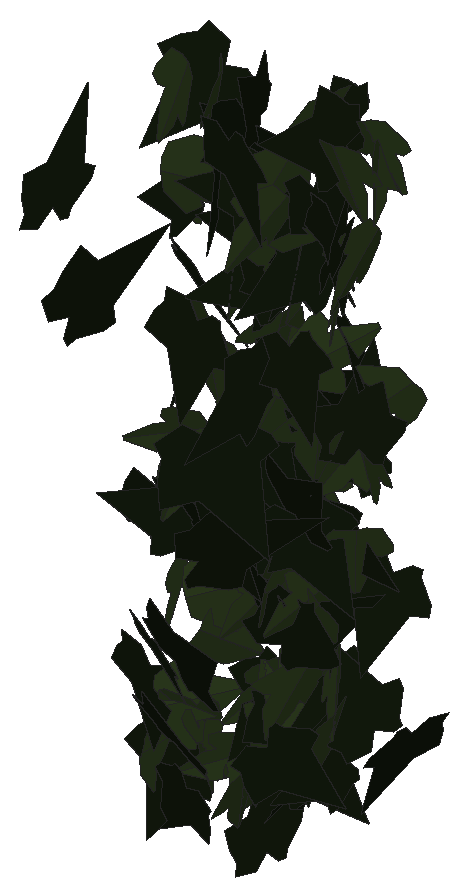
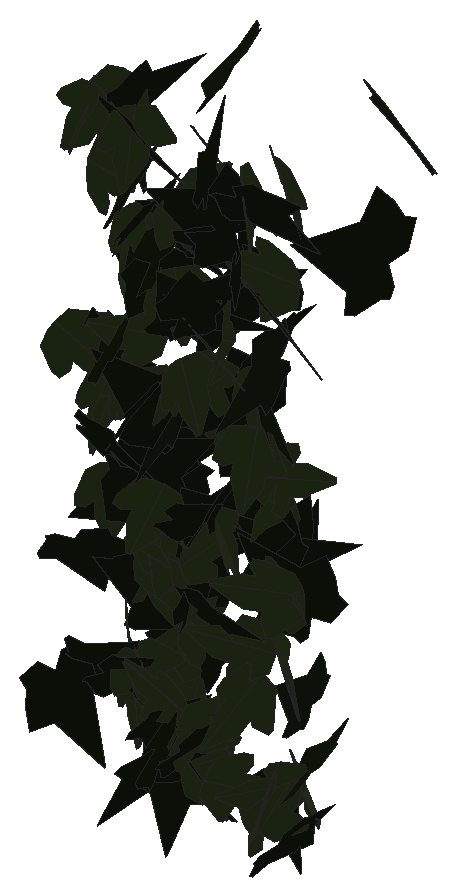
# SketchUp Ruby script. Lengths in inches.
U = 1.inch
M = Sketchup.active_model
def pt(a) = Geom::Point3d.new(a.map { |v| v * U })
def face(e, loops, mat)
  f = e.add_face(loops[0].map { |a| pt(a) })
  loops[1..].each { |l| e.add_face(l.map { |a| pt(a) }).erase! }
  f.material = f.back_material = mat if mat
  f
end
# faces: each face lists its corners as indices into pts; further lists are holes
def faces(e, pts, list, mat = nil) = list.each { |f| face(e, (f[0].is_a?(Array) ? f : [f]).map { |l| l.map { |i| pts[i] } }, mat) }
# xy, xz, yz: faces in a plane at the given z, y or x. An outline is a flat list of corners, or four numbers for a rectangle; further outlines are holes
def ring(l) = l.size == 4 ? [[l[0], l[1]], [l[2], l[1]], [l[2], l[3]], [l[0], l[3]]] : l.each_slice(2).to_a
def flat(e, list, mat, &to3) = list.each { |f| face(e, (f[0].is_a?(Array) ? f : [f]).map { |l| ring(l).map { |u, v| to3.(u, v) } }, mat) }
def xy(e, z, list, mat = nil) = flat(e, list, mat) { |x, y| [x, y, z] }
def xz(e, y, list, mat = nil) = flat(e, list, mat) { |x, z| [x, y, z] }
def yz(e, x, list, mat = nil) = flat(e, list, mat) { |y, z| [x, y, z] }
def lines(e, pts, list) = list.each { |a, b| e.add_line(pt(pts[a]), pt(pts[b])) }
# prism: a flat outline (further loops are holes) pulled along v
def prism(e, loops, v, mat = nil)
  f = face(e, loops, mat); d = Geom::Vector3d.new(v.map { |x| x * U })
  f.pushpull(f.normal.samedirection?(d) ? d.length : -d.length)
end
def box(e, o, s, mat = nil) = prism(e, [[o, [o[0] + s[0], o[1], o[2]], [o[0] + s[0], o[1] + s[1], o[2]], [o[0], o[1] + s[1], o[2]]]], [0, 0, s[2]], mat)
def at(x, y, z, deg = 0) = Geom::Transformation.translation(pt([x, y, z])) * Geom::Transformation.rotation(ORIGIN, Z_AXIS, deg.degrees)
def axes(o, x, y, z) = Geom::Transformation.new([*x, 0, *y, 0, *z, 0, *pt(o).to_a, 1])
def part(name) = M.definitions.add(name)
# library, detail: a bought-in or finely detailed component or shape, given as its bounding box
def library(name, o, s) = part(name).tap { |d| box(d.entities, o, s) }
def detail(e, o, s) = box(e.add_group.entities, o, s)
def put(e, d, t, mat = nil) = e.add_instance(d, t).tap { |i| i.material = mat if mat }
def group(e, t, mat = nil) = e.add_group.tap { |g| g.transformation = t; g.material = mat if mat }.entities
root = M.entities
M.materials.add("efeu1").color = [18, 25, 13]
M.materials.add("efeu2").color = [43, 57, 29]
c1 = part("ivyleaf_9")
p = [[1.54,2.16,1.25],[1.36,2.04,1.19],[-0.21,0.99,0.68],[-0.71,1.11,0.82],[-0.85,0.86,0.67],[-0.8,0.17,0.21],
  [-0.9,-0.01,0.1],[-0.67,-0.16,-0.02],[-0.08,-0.08,-0.05],[-0.03,-0.6,-0.4],[0.65,-0.88,-0.66],[0.83,-0.6,-0.49],
  [1.29,-0.42,-0.43],[1.8125,-0.07,-0.26],[1.21,0.44,0.15]]
faces(c1.entities,p,[[0,1,2,3,4,5,6,7,8,9,10,11,12,13,14]],"efeu1")
c2 = part("ivyleaf_10")
p = [[0,0.5,-0.03],[-0.0625,2.02,-0.43],[-0.19,2.01,-0.46],[-0.54,1.05,-0.29],[-0.52,0.625,-0.18],[-0.83,0.76,-0.28],
  [-1.16,0.64,-0.33],[-1.15,0.33,-0.24],[-0.77,-0.39,0.02],[-0.3,-0.51,0.16],[0.04,-0.48,0.23],[-0.02,2.01,-0.4375],
  [-0.06,2.01,-0.43],[0.04,-0.49,0.23],[0.67,-0.49,0.14],[1.38,0.36,-0.2],[1.375,0.51,-0.24],[0.81,0.65,-0.19],
  [0.62,0.59,-0.15],[0.6,1.09,-0.28],[0.5,1.23,-0.31]]
faces(c2.entities,p,[[0,1,2,3,4,5,6,7,8,9,10],[11,12,0,13,14,15,16,17,18,19,20]],"efeu2")
put(root,c1,axes([542.46,125.34,201.33],[-0.99662,0.33655,-0.15122],[0.14199,-0.05215,-1.05191],[-0.34055,-1.00668,0.00394]))
put(root,c1,axes([538.84,126.51,189.16],[0.8472,-0.56615,0.10588],[-0.08782,0.05915,1.01896],[-0.56923,-0.85174,0.00038]))
put(root,c1,axes([535.7,125.54,204.25],[-0.88917,0.67387,-0.10406],[-0.08581,0.05905,1.11567],[0.67644,0.89329,0.00475]))
put(root,c1,axes([540.1875,126.3,198.45],[-0.02484,-0.85792,-0.79296],[0.14605,0.78464,-0.85349],[1.15909,-0.11726,0.09055]))
put(root,c1,axes([538.32,127.29,190.98],[-0.04579,-0.29377,1.10403],[0.68746,-0.88957,-0.20819],[0.91246,0.65547,0.21226]))
put(root,c1,axes([535.68,126.37,200.66],[0.09702,0.07319,1.16134],[0.78915,0.8523,-0.11964],[-0.85517,0.7948,0.02135]))
put(root,c1,axes([539.65,126.72,194.68],[0.39362,0.23601,1.0665],[0.91867,0.54173,-0.45895],[-0.5909,0.99945,-0.00309]))
put(root,c1,axes([539.36,128.17,206.05],[0.42505,-0.88524,0.22608],[0.10685,-0.19947,-0.98195],[0.90738,0.43817,0.00972]))
put(root,c1,axes([540.29,128.63,188.47],[0.02358,-0.21935,-0.82404],[0.27211,0.78319,-0.20069],[0.80815,-0.25731,0.09162]))
put(root,c2,axes([539.11,128.93,187.01],[0.06972,-0.81984,-0.18916],[-0.01731,0.18837,-0.8228],[0.8412,0.07183,-0.00125]))
put(root,c1,axes([540.54,129.16,200.02],[0.08511,-0.8096,-0.26487],[-0.02314,0.26389,-0.81405],[0.85151,0.08809,0.00435]))
put(root,c1,axes([536.93,129.78,199.24],[-0.02769,-0.95204,0.27297],[-0.01795,-0.27255,-0.95239],[0.99024,-0.03156,-0.00964]))
put(root,c1,axes([536.92,129.39,185.79],[0.32793,0.12421,-0.75032],[-0.71071,-0.24082,-0.35049],[-0.27073,0.78264,0.01124]))
put(root,c1,axes([540.08,129.92,194.74],[-0.28154,-0.08244,0.94768],[0.58247,-0.79632,0.10377],[0.75208,0.58587,0.27439]))
put(root,c1,axes([542,128.98,203.02],[0.13248,0.21807,0.82631],[-0.1013,0.83429,-0.20394],[-0.84858,-0.06555,0.15335]))
put(root,c2,axes([539.08,130.26,203.14],[-0.12291,-0.64575,0.69785],[-0.04154,-0.69934,-0.65444],[0.94988,-0.11414,0.06168]))
put(root,c2,axes([542.03,130.39,203.1],[0.14763,-0.60488,0.75555],[0.23882,-0.71789,-0.62139],[0.93792,0.278,0.0393]))
put(root,c2,axes([539.28,129.92,197.56],[-0.67822,-0.56031,0.38123],[-0.30162,-0.23343,-0.87966],[0.60688,-0.74218,-0.01114]))
put(root,c2,axes([535.17,130.08,186.01],[0.2974,-0.46163,-0.60165],[0.44807,-0.41442,0.53946],[-0.61181,-0.5279,0.10262]))
put(root,c1,axes([535.17,130.17,189.2],[0.36127,-0.5464,0.48417],[0.28485,-0.39189,-0.65481],[0.67218,0.45974,0.01727]))
put(root,c2,axes([536.34,130.23,194.875],[0.1111,0.59983,-0.55383],[-0.11032,-0.54278,-0.60999],[-0.80892,0.15641,0.00713]))
put(root,c1,axes([538.37,130.21,193.11],[0.34532,0.16862,0.86839],[-0.84103,-0.22643,0.3784],[0.27425,-0.90669,0.06699]))
put(root,c1,axes([536.37,130.16,193.15],[-0.29124,0.00633,0.77085],[-0.76742,-0.08043,-0.28928],[0.07301,-0.8201,0.03432]))
put(root,c2,axes([536.35,130.28,195.69],[0.01568,0.15758,-0.80777],[-0.7282,-0.37377,-0.08705],[-0.38345,0.71626,0.13228]))
put(root,c2,axes([539.22,130.32,193.16],[0.47656,-0.76573,0.36457],[0.19543,-0.30778,-0.90191],[0.82527,0.51506,0.00305]))
put(root,c1,axes([539.44,129.54,184.93],[-0.8793,0.36104,-0.12202],[-0.12025,0.02832,0.95034],[0.36163,0.88728,0.01932]))
put(root,c1,axes([540.16,129.96,194.58],[-0.21178,-0.51876,-0.81864],[0.42013,0.70598,-0.55606],[0.87336,-0.46541,0.06898]))
put(root,c1,axes([538.51,129.92,196.47],[0.03525,-0.68505,-0.71505],[0.12812,0.71265,-0.67643],[0.98192,-0.0684,0.11393]))
put(root,c1,axes([540.95,130.74,205.49],[-0.29247,-0.1571,0.84291],[-0.55236,-0.64666,-0.31218],[0.65581,-0.61471,0.11298]))
put(root,c2,axes([540.11,130.67,192.11],[-0.02903,-0.37937,0.73832],[-0.07834,-0.73422,-0.38035],[0.82638,-0.08293,-0.01012]))
put(root,c1,axes([535.86,130.36,193.2],[0.22248,-0.24255,0.75106],[0.55341,-0.50842,-0.32813],[0.56272,0.5959,0.02575]))
put(root,c1,axes([540.43,130.4,202.18],[-0.96021,-0.022,0.11467],[-0.11468,-0.00107,-0.96046],[0.02197,-0.96704,-0.00155]))
put(root,c2,axes([538.55,130.81,186.38],[0.02886,-0.1984,0.87429],[0.28414,-0.82763,-0.19719],[0.8503,0.2833,0.03622]))
put(root,c1,axes([540.74,130.7,202.98],[0.25081,-0.78857,0.41667],[0.09233,-0.40755,-0.82689],[0.88709,0.26538,-0.03174]))
put(root,c2,axes([541.44,130.12,205.51],[-0.91099,0.12476,-0.14051],[0.13928,-0.01856,-0.91949],[-0.12613,-0.92158,-0.0005]))
put(root,c2,axes([539.56,130.68,189.38],[-0.2199,-0.7841,0.39939],[-0.0943,-0.3883,-0.81425],[0.87489,-0.23893,0.01262]))
put(root,c2,axes([541.32,130.85,196.67],[0.12495,0.40976,-0.73646],[-0.27603,-0.68354,-0.42715],[-0.79629,0.30125,0.03251]))
put(root,c1,axes([541.21,130.47,187.64],[-0.8341,0.23111,0.14881],[-0.14103,0.04828,-0.86548],[-0.23593,-0.84589,-0.00874]))
put(root,c1,axes([534.47,131,187.76],[0.11316,-0.82051,0.52307],[0.19804,-0.49615,-0.82113],[0.95269,0.2006,0.10856]))
put(root,c1,axes([539.625,130.11,190.76],[0.03089,-0.03752,1.01668],[1.01548,0.06315,-0.02852],[-0.06202,1.01518,0.03935]))
put(root,c1,axes([537.82,130.85,191.59],[0.18788,-0.24664,0.81519],[0.45505,-0.67658,-0.30958],[0.71993,0.49202,-0.01706]))
put(root,c2,axes([539.84,130.4,193.28],[-0.12617,-0.83042,-0.28085],[0.08315,0.27113,-0.83902],[0.87267,-0.1459,0.03934]))
put(root,c2,axes([539.41,131.1,201.29],[-0.12043,0.36573,-0.84418],[0.15735,-0.83065,-0.38231],[-0.90644,-0.19278,0.04579]))
put(root,c2,axes([540.24,130.52,191.7],[-0.6008,-0.09231,0.56672],[-0.56344,-0.06319,-0.60761],[0.11059,-0.82349,-0.0169]))
put(root,c2,axes([540.73,130.54,188.48],[0.09044,-1.00171,-0.21244],[-0.01562,0.21189,-1.00578],[1.02387,0.09171,0.00342]))
put(root,c2,axes([540.3125,130.64,197.17],[-0.54331,-0.75573,0.04251],[-0.02497,-0.0344,-0.93076],[0.75651,-0.54389,-0.0002]))
put(root,c2,axes([537.52,130.9375,186.35],[0.17737,0.20389,-0.77068],[-0.69886,-0.3401,-0.25081],[-0.38356,0.71396,0.10061]))
put(root,c1,axes([541.83,130.34,197.22],[-0.86554,0.12266,0.31],[0.30628,-0.04806,0.87418],[0.13167,0.91812,0.00434]))
put(root,c1,axes([534.81,130.67,192.28],[-0.08917,-0.08834,0.95115],[0.88508,-0.367,0.04889],[0.35935,0.88201,0.11561]))
put(root,c2,axes([535.52,130.875,190.81],[0.60911,-0.71971,0.06776],[0.03552,-0.05871,-0.94281],[0.72202,0.61005,-0.01078]))
put(root,c2,axes([540.23,130.79,202.3125],[-0.65535,-0.57392,0.21737],[-0.16971,-0.13612,-0.87109],[0.58977,-0.67691,-0.00913]))
put(root,c1,axes([535.16,131.4,185.51],[-0.19084,-0.88951,0.3733],[-0.03711,-0.37348,-0.90892],[0.96395,-0.19048,0.03891]))
put(root,c2,axes([541.39,130.75,194.05],[-0.59206,-0.6106,0.00529],[-0.00253,-0.00492,-0.85051],[0.61062,-0.59207,0.00161]))
put(root,c1,axes([536.01,131.02,198.15],[-0.53846,0.23639,-0.57178],[0.51667,-0.24522,-0.58794],[-0.34039,-0.74615,0.01208]))
put(root,c2,axes([538.84,130.66,187.8],[0.76337,0.14221,0.28272],[-0.28874,0.01077,0.77421],[0.12955,-0.81397,0.05964]))
put(root,c2,axes([541.91,131.14,205.21],[-0.13866,0.6043,-0.58634],[0.13734,-0.57005,-0.61999],[-0.83073,-0.19511,-0.00463]))
put(root,c2,axes([535.47,130.91,205.46],[0.8037,-0.57535,-0.12169],[-0.09929,0.07036,-0.98841],[0.57964,0.80981,-0.00058]))
put(root,c2,axes([540.29,131.21,189.77],[0.59005,-0.40846,0.58896],[0.49745,-0.31582,-0.71741],[0.516,0.77155,0.01814]))
put(root,c2,axes([537.97,131.41,191.1],[-0.09927,-0.47209,0.65973],[-0.1036,-0.65183,-0.48203],[0.8046,-0.14218,0.01934]))
put(root,c1,axes([540.22,130.74,194.24],[-0.03418,0.0148,-0.93069],[0.70498,0.60852,-0.01621],[0.60778,-0.70501,-0.03353]))
put(root,c2,axes([536.6,130.78,198.625],[-0.69296,0.28336,0.34939],[-0.35142,0.05958,-0.74533],[-0.28083,-0.77377,0.07056]))
put(root,c2,axes([540.24,131.55,200.87],[0.25906,-0.25932,0.86648],[0.60434,-0.62095,-0.36653],[0.67291,0.65751,-0.0044]))
put(root,c1,axes([538.31,131.4,200.36],[-0.66785,-0.07874,0.49317],[-0.4654,-0.20058,-0.66228],[0.18115,-0.80561,0.11669]))
put(root,c2,axes([541.61,130.88,196.7],[-0.7708,0.32663,0.14969],[-0.13575,0.0633,-0.83713],[-0.33266,-0.78264,-0.00523]))
put(root,c1,axes([539.4375,130.6,185.9],[-0.00005,0.82108,0.13207],[0.0001,0.13207,-0.82108],[-0.83163,-0.00004,-0.0001]))
put(root,c1,axes([539.95,131.17,195.07],[0.00198,0.04985,0.84064],[-0.82411,0.17301,-0.00832],[-0.1732,-0.82265,0.04919]))
put(root,c2,axes([535.99,131.45,185.83],[-0.04453,-0.04414,-0.80849],[0.55456,-0.59165,0.00176],[-0.58997,-0.5528,0.06267]))
put(root,c1,axes([536.4,131.6,203.11],[-0.10596,0.03786,-0.92487],[0.80515,-0.4555,-0.11089],[-0.45667,-0.81187,0.01908]))
put(root,c1,axes([538.09,131.73,191.45],[-0.06528,-0.10747,0.81775],[-0.34564,-0.74124,-0.12501],[0.74887,-0.35148,0.01359]))
put(root,c2,axes([542.25,131.49,198.43],[-0.4109,-0.37972,0.66855],[-0.45696,-0.48901,-0.5586],[0.61833,-0.61372,0.03145]))
put(root,c1,axes([538.83,131.35,188.11],[-0.08597,-0.83193,-0.3462],[0.04587,0.34328,-0.83631],[0.89992,-0.09698,0.00956]))
put(root,c2,axes([535.47,131.58,186.28],[-0.51546,-0.38488,-0.46913],[-0.29799,-0.37564,0.63561],[-0.5286,0.58709,0.09914]))
put(root,c2,axes([539.19,131.46,192.59],[-0.14517,-0.09052,-0.81757],[0.69592,-0.45612,-0.07307],[-0.43853,-0.69386,0.15469]))
put(root,c1,axes([541.64,131.09,188.5625],[-0.85608,-0.23087,-0.17692],[-0.17114,-0.04484,0.88667],[-0.23518,0.87302,-0.00125]))
put(root,c2,axes([535,131.25,192.85],[0.29861,0.02888,0.8239],[0.8194,0.08607,-0.3],[-0.09075,0.87211,0.00232]))
put(root,c2,axes([538.39,131.54,203.61],[-0.42619,-0.66346,0.40932],[-0.16112,-0.38146,-0.78606],[0.76273,-0.45129,0.06267]))
put(root,c2,axes([535.23,131.26,202.43],[0.02868,0.00345,-0.99141],[0.97443,-0.18293,0.02755],[-0.18276,-0.97481,-0.00868]))
put(root,c2,axes([540,130.71,198.88],[0.24452,0.18388,-0.87899],[0.6528,0.58919,0.30485],[0.61668,-0.69662,0.02583]))
put(root,c2,axes([538.41,131.48,192.17],[-0.44053,0.17875,-0.66675],[0.52945,-0.42003,-0.46243],[-0.44293,-0.67985,0.11039]))
put(root,c2,axes([536.32,130.91,190.74],[0.25068,0.06473,-0.91337],[0.85418,0.3246,0.25744],[0.32985,-0.88978,0.02747]))
put(root,c1,axes([537.91,131.5,202.59],[-0.51409,0.14637,0.63984],[-0.65575,-0.07931,-0.50873],[-0.02845,-0.81694,0.16403]))
put(root,c2,axes([536.8,131.8,200.36],[-0.10887,0.51045,-0.77588],[0.17262,-0.75646,-0.52189],[-0.91255,-0.20399,-0.00616]))
put(root,c1,axes([539.52,131.45,203.27],[0.3723,-0.80605,-0.21126],[-0.05274,0.20813,-0.88705],[0.8316,0.37406,0.03832]))
put(root,c1,axes([537.09,132.13,194.93],[-0.05707,-0.68672,0.7197],[-0.04583,-0.7183,-0.68902],[0.9937,-0.07257,0.00955]))
put(root,c1,axes([539.01,131.77,201.95],[0.48385,-0.67927,0.51897],[0.33871,-0.39519,-0.83304],[0.78487,0.58929,0.03957]))
put(root,c2,axes([539.83,131.51,189.47],[-0.60602,-0.43763,0.38033],[-0.3131,-0.21605,-0.74749],[0.488,-0.68209,-0.00726]))
put(root,c1,axes([537.35,131.85,204.66],[-0.03865,0.26157,0.84229],[-0.19619,-0.82453,0.24705],[0.85987,-0.17637,0.09423]))
put(root,c1,axes([539.35,131.29,197.8],[0.44338,-0.66642,-0.42409],[-0.11999,0.42387,-0.79152],[0.78075,0.4436,0.1192]))
put(root,c2,axes([538.59,131.49,201.23],[-0.54218,-0.61606,0.11639],[-0.06767,-0.09547,-0.82057],[0.62329,-0.54625,0.01215]))
put(root,c2,axes([537.87,131.88,188.22],[0.14568,0.38897,-0.73894],[-0.42404,-0.61174,-0.40561],[-0.71939,0.43935,0.08945]))
put(root,c1,axes([535.37,131.27,199.9375],[0.89643,-0.3728,-0.19959],[-0.17735,0.09323,-0.9707],[0.38388,0.91364,0.01761]))
put(root,c2,axes([538.4375,131.72,198.37],[-0.00235,0.68767,-0.46304],[-0.10045,-0.45986,-0.68245],[-0.82292,0.05417,0.08463]))
put(root,c1,axes([540.54,131.95,189.01],[-0.60682,-0.40056,0.3226],[-0.27909,-0.16263,-0.72691],[0.432,-0.66772,-0.01648]))
put(root,c1,axes([539.22,131.66,201.59],[-0.12917,0.55464,-0.60963],[0.13295,-0.59497,-0.56947],[-0.81339,-0.18533,0.00373]))
put(root,c2,axes([536.46,130.97,189.54],[-0.20919,-0.57342,-0.79102],[0.36114,0.70627,-0.60749],[0.9078,-0.41311,0.05939]))
put(root,c2,axes([541.42,131.43,205.64],[-0.76845,0.12602,-0.35686],[0.34936,-0.0744,-0.77857],[-0.14554,-0.844,0.01534]))
put(root,c1,axes([538.81,131.46,196.99],[0.0321,-0.14683,0.97769],[0.943,-0.28929,-0.07441],[0.29698,0.93447,0.13059]))
put(root,c1,axes([541.64,131.88,192.59],[-0.60016,-0.65943,-0.19569],[0.13351,0.1431,-0.89165],[0.67478,-0.61483,0.00236]))
put(root,c2,axes([537.5,132.08,193.55],[-0.08138,0.21723,0.77842],[0.05773,-0.77879,0.22337],[0.8061,0.07771,0.06259]))
put(root,c1,axes([537.79,132.24,187.77],[-0.32497,-0.71147,0.46147],[-0.14543,-0.44012,-0.78096],[0.83546,-0.35336,0.04356]))
put(root,c1,axes([538.45,131.375,200.24],[-0.65719,0.53031,0.365],[-0.30066,0.2084,-0.84411],[-0.56926,-0.72229,0.02444]))
put(root,c2,axes([536.76,131.79,194.54],[0.38026,-0.70038,0.1872],[0.08818,-0.16514,-0.79695],[0.71959,0.39035,-0.00127]))
put(root,c1,axes([540.62,131.5625,205.59],[-0.75895,0.34085,0.31775],[-0.28014,0.15154,-0.83168],[-0.37238,-0.8087,-0.02193]))
put(root,c2,axes([535.22,130.99,187.06],[0.21572,-0.12873,-0.94919],[0.6701,0.71553,0.05525],[0.68447,-0.65993,0.24506]))
put(root,c1,axes([538.63,131.4,197.42],[0.6855,-0.264,-0.36948],[-0.33741,0.15167,-0.73435],[0.30392,0.76382,0.01811]))
put(root,c1,axes([540.36,132.19,198.66],[0.05336,-0.47697,0.67741],[0.19013,-0.65364,-0.47521],[0.80637,0.18569,0.06722]))
put(root,c2,axes([538.05,131.79,198.81],[-0.23674,-0.80112,0.11737],[-0.04656,-0.10861,-0.83525],[0.80833,-0.24088,-0.01374]))
put(root,c1,axes([542.39,131.74,188.24],[-0.27184,0.74942,-0.55981],[0.13591,-0.54514,-0.79577],[-0.92549,-0.30018,0.04756]))
put(root,c1,axes([538.05,132.16,194.6],[-0.6588,-0.31045,0.38865],[-0.33308,-0.20371,-0.72733],[0.36944,-0.73727,0.03731]))
put(root,c1,axes([538.55,132.29,187.28],[0.19412,-0.49314,0.77936],[0.27552,-0.72906,-0.52994],[0.88016,0.33698,-0.00601]))
put(root,c1,axes([536.51,131.75,203.7],[0.42107,-0.18618,0.85758],[0.79142,-0.33041,-0.46032],[0.37916,0.89643,0.00844]))
put(root,c2,axes([534.9375,131.55,193.18],[-0.01127,-0.10949,-0.99075],[0.9893,0.11993,-0.0245],[0.12189,-0.98353,0.10731]))
put(root,c2,axes([536.1,131.68,205.2],[0.3764,-0.77323,-0.24016],[-0.0431,0.24533,-0.85743],[0.80852,0.37305,0.06609]))
put(root,c1,axes([538.3,131.4,200.24],[-0.40948,-0.26051,0.67771],[0.5484,0.39895,0.4847],[-0.47583,0.68397,-0.02459]))
put(root,c2,axes([535.91,131.68,197.39],[-0.92776,-0.00435,0.0386],[-0.03859,-0.00217,-0.92776],[0.00444,-0.92856,0.00198]))
put(root,c1,axes([539.15,131.52,186.63],[0.22237,-0.48451,-0.67386],[-0.03779,0.691,-0.5093],[0.8291,0.16144,0.15752]))
put(root,c2,axes([538.57,131.8,188.78],[0.40954,-0.11452,-0.71294],[0.70776,-0.09875,0.42243],[-0.14308,-0.81624,0.04892]))
put(root,c1,axes([541.2,131.88,196.09],[-0.7203,0.18837,0.3015],[-0.28526,0.10028,-0.74417],[-0.21215,-0.77439,-0.02303]))
put(root,c2,axes([539.1,131.71,194.68],[-0.75139,-0.2407,-0.27073],[0.25957,0.07712,-0.78898],[0.25269,-0.79494,0.00544]))
put(root,c1,axes([537.6,131.71,191.85],[-0.38874,0.35747,0.62926],[-0.58057,0.27243,-0.51342],[-0.43209,-0.68766,0.12371]))
put(root,c2,axes([535.54,131.78,186.25],[-0.32734,0.73544,-0.06457],[-0.06049,0.04367,0.80413],[0.73579,0.33078,0.03738]))
put(root,c1,axes([537.625,132.45,201.02],[-0.15235,-0.06419,0.88028],[-0.70979,-0.52204,-0.16091],[0.52461,-0.72496,0.03793]))
put(root,c2,axes([539.79,131.8,205.79],[-0.41498,-0.78058,-0.19292],[0.08689,0.1723,-0.88402],[0.79936,-0.42396,-0.00406]))
put(root,c1,axes([535.49,131.7,201.82],[-0.6388,0.56264,0.37307],[-0.2927,0.232,-0.85107],[-0.60834,-0.70244,0.01773]))
put(root,c1,axes([535.7,132.37,205.18],[-0.94211,-0.33008,0.09395],[-0.0842,-0.04378,-0.99817],[0.3327,-0.94577,0.01342]))
